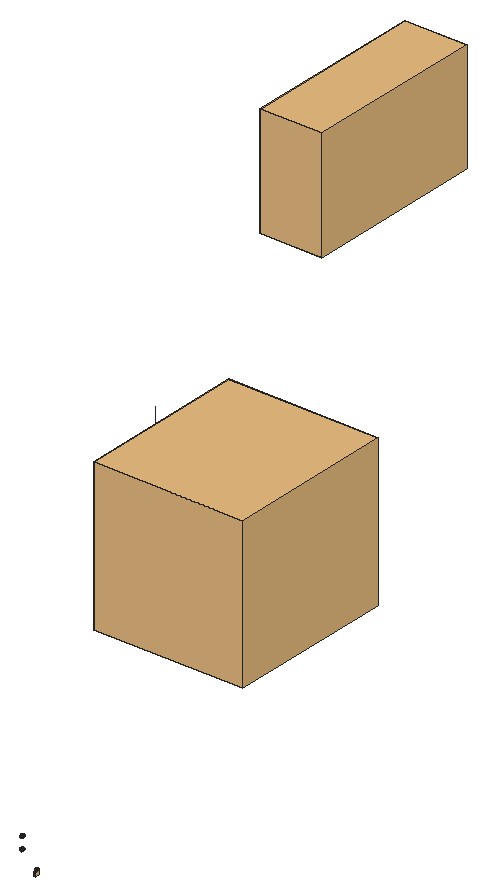
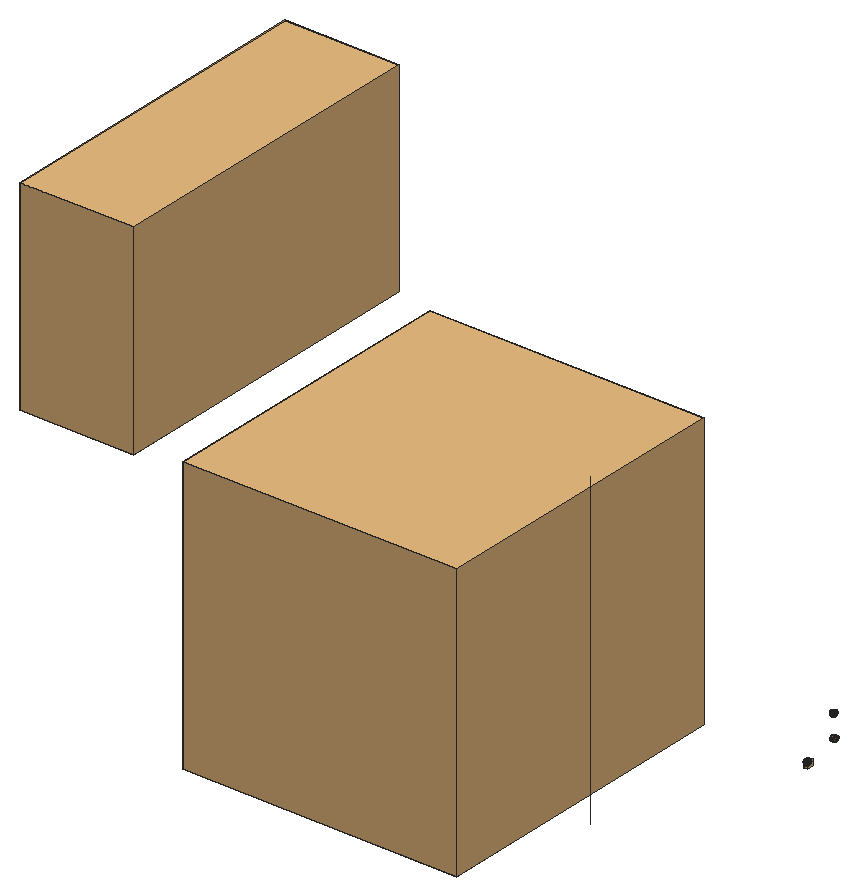
# SketchUp Ruby script. Lengths in inches.
U = 1.inch
M = Sketchup.active_model
def pt(a) = Geom::Point3d.new(a.map { |v| v * U })
def face(e, loops, mat)
  f = e.add_face(loops[0].map { |a| pt(a) })
  loops[1..].each { |l| e.add_face(l.map { |a| pt(a) }).erase! }
  f.material = f.back_material = mat if mat
  f
end
# faces: each face lists its corners as indices into pts; further lists are holes
def faces(e, pts, list, mat = nil) = list.each { |f| face(e, (f[0].is_a?(Array) ? f : [f]).map { |l| l.map { |i| pts[i] } }, mat) }
# xy, xz, yz: faces in a plane at the given z, y or x. An outline is a flat list of corners, or four numbers for a rectangle; further outlines are holes
def ring(l) = l.size == 4 ? [[l[0], l[1]], [l[2], l[1]], [l[2], l[3]], [l[0], l[3]]] : l.each_slice(2).to_a
def flat(e, list, mat, &to3) = list.each { |f| face(e, (f[0].is_a?(Array) ? f : [f]).map { |l| ring(l).map { |u, v| to3.(u, v) } }, mat) }
def xy(e, z, list, mat = nil) = flat(e, list, mat) { |x, y| [x, y, z] }
def xz(e, y, list, mat = nil) = flat(e, list, mat) { |x, z| [x, y, z] }
def yz(e, x, list, mat = nil) = flat(e, list, mat) { |y, z| [x, y, z] }
def lines(e, pts, list) = list.each { |a, b| e.add_line(pt(pts[a]), pt(pts[b])) }
# prism: a flat outline (further loops are holes) pulled along v
def prism(e, loops, v, mat = nil)
  f = face(e, loops, mat); d = Geom::Vector3d.new(v.map { |x| x * U })
  f.pushpull(f.normal.samedirection?(d) ? d.length : -d.length)
end
def box(e, o, s, mat = nil) = prism(e, [[o, [o[0] + s[0], o[1], o[2]], [o[0] + s[0], o[1] + s[1], o[2]], [o[0], o[1] + s[1], o[2]]]], [0, 0, s[2]], mat)
def at(x, y, z, deg = 0) = Geom::Transformation.translation(pt([x, y, z])) * Geom::Transformation.rotation(ORIGIN, Z_AXIS, deg.degrees)
def axes(o, x, y, z) = Geom::Transformation.new([*x, 0, *y, 0, *z, 0, *pt(o).to_a, 1])
def part(name) = M.definitions.add(name)
# library, detail: a bought-in or finely detailed component or shape, given as its bounding box
def library(name, o, s) = part(name).tap { |d| box(d.entities, o, s) }
def detail(e, o, s) = box(e.add_group.entities, o, s)
def put(e, d, t, mat = nil) = e.add_instance(d, t).tap { |i| i.material = mat if mat }
def group(e, t, mat = nil) = e.add_group.tap { |g| g.transformation = t; g.material = mat if mat }.entities
root = M.entities
M.materials.add("green").color = [174, 139, 102]
M.materials.add("vio").color = [206, 114, 100]
c1 = part("3DGeom~232_Defintion")
p = [[-0.24,-111.46,-482.48],[-247.71,40.8125,-431.68],[-3.37,-2.64,-500],[241.88,-45.39,-434.35],[50.53,96.35,-484.34],[-154.36,212.27,-404.56],
  [147.01,158.99,-439.69],[12.76,320.76,-327.23],[59.09,-200.9375,-436.46],[-242.29,-147.66,-401.33],[260.24,168.49,-378.02],[208.87,337.23,-220.41],
  [208.87,337.23,-220.41],[-139.53,-302.65,-321.625],[158.71,-247.11,-374.29],[271.93,-237.61,-312.62],[368.42,-174.96,-267.97],[422.32,-75.98,-252.31],
  [419.18,32.84,-269.83],[359.86,122.32,-315.85],[-242.29,-147.66,-401.33],[-425.69,73.33,-247.69],[-247.71,40.8125,-431.68],[-425.69,73.33,-247.69],
  [-317.89,271.31,-216.375],[-317.89,271.31,-216.375],[-154.36,212.27,-404.56],[-317.89,271.31,-216.375],[-124.92,396.59,-127.08],[-154.36,212.27,-404.56],
  [12.76,320.76,-327.23],[-139.53,-302.65,-321.625],[-419.42,-144.29,-212.64],[-242.29,-147.66,-401.33],[-242.29,-147.66,-401.33],[-425.69,73.33,-247.69],
  [260.24,168.49,-378.02],[381.41,257.26,-112.72],[359.86,122.32,-315.85],[260.24,168.49,-378.02],[208.87,337.23,-220.41],[33.01,-382.62,-213.94],
  [271.93,-237.61,-312.62],[33.01,-382.62,-213.94],[158.71,-247.11,-374.29],[12.76,320.76,-327.23],[101.53,415.61,-3.73],[12.76,320.76,-327.23],
  [208.87,337.23,-220.41],[33.01,-382.62,-213.94],[-300.77,-323.26,-120.61],[-139.53,-302.65,-321.625],[-139.53,-302.65,-321.625],[-300.77,-323.26,-120.61],
  [359.86,122.32,-315.85],[484.17,102.27,-33.02],[419.18,32.84,-269.83],[359.86,122.32,-315.85],[271.93,-237.61,-312.62],[229.12,-366.15,-107.12],
  [33.01,-382.62,-213.94],[368.42,-174.96,-267.97],[229.12,-366.15,-107.12],[271.93,-237.61,-312.62],[419.18,32.84,-269.83],[489.59,-86.2,-2.67],
  [419.18,32.84,-269.83],[422.32,-75.98,-252.31],[368.42,-174.96,-267.97],[396.24,-257.66,-29.79],[229.12,-366.15,-107.12],[422.32,-75.98,-252.31],
  [368.42,-174.96,-267.97],[422.32,-75.98,-252.31],[-489.59,86.2,2.67],[-425.69,73.33,-247.69],[-425.69,73.33,-247.69],[-396.24,257.66,29.79],
  [-425.69,73.33,-247.69],[-396.24,257.66,29.79],[-317.89,271.31,-216.375],[208.87,337.23,-220.41],[300.77,323.26,120.61],[381.41,257.26,-112.72],
  [208.87,337.23,-220.41],[300.77,323.26,120.61],[-396.24,257.66,29.79],[-229.12,366.15,107.12],[33.01,-382.62,-213.94],[-101.53,-415.61,3.73],
  [-300.77,-323.26,-120.61],[33.01,-382.62,-213.94],[-484.17,-102.27,33.02],[-33.01,382.62,213.94],[-381.41,-257.26,112.72],[-300.77,-323.26,-120.61],
  [-381.41,-257.26,112.72],[419.42,144.29,212.64],[300.77,323.26,120.61],[124.92,-396.59,127.08],[396.24,-257.66,-29.79],[425.69,-73.33,247.69],
  [396.24,-257.66,-29.79],[317.89,-271.31,216.375],[317.89,-271.31,216.375],[139.53,302.65,321.625],[139.53,302.65,321.625],[300.77,323.26,120.61],
  [-422.32,75.98,252.31],[-368.42,174.96,267.97],[-396.24,257.66,29.79],[-208.87,-337.23,220.41],[-381.41,-257.26,112.72],[-396.24,257.66,29.79],
  [-271.93,237.61,312.62],[-396.24,257.66,29.79],[-271.93,237.61,312.62],[-229.12,366.15,107.12],[-419.18,-32.84,269.83],[-271.93,237.61,312.62],
  [-158.71,247.11,374.29],[-158.71,247.11,374.29],[-208.87,-337.23,220.41],[-359.86,-122.32,315.85],[242.29,147.66,401.33],[139.53,302.65,321.625],
  [-12.76,-320.76,327.23],[317.89,-271.31,216.375],[247.71,-40.8125,431.68],[247.71,-40.8125,431.68],[-33.01,382.62,213.94],[-158.71,247.11,374.29],
  [-59.09,200.94,436.46],[-33.01,382.62,213.94],[139.53,302.65,321.625],[317.89,-271.31,216.375],[154.36,-212.27,404.56],[425.69,-73.33,247.69],
  [154.36,-212.27,404.56],[317.89,-271.31,216.375],[-208.87,-337.23,220.41],[-260.24,-168.49,378.02],[-12.76,-320.76,327.23],[-260.24,-168.49,378.02],
  [-208.87,-337.23,220.41],[425.69,-73.33,247.69],[247.71,-40.8125,431.68],[-422.32,75.98,252.31],[-419.18,-32.84,269.83],[-241.88,45.39,434.35],
  [-368.42,174.96,267.97],[-422.32,75.98,252.31],[-271.93,237.61,312.62],[-368.42,174.96,267.97],[-419.18,-32.84,269.83],[-359.86,-122.32,315.85],
  [-271.93,237.61,312.62],[-359.86,-122.32,315.85],[-260.24,-168.49,378.02],[139.53,302.65,321.625],[0.24,111.46,482.48],[139.53,302.65,321.625],
  [242.29,147.66,401.33],[-12.76,-320.76,327.23],[-147.01,-158.99,439.69],[-260.24,-168.49,378.02],[-12.76,-320.76,327.23],[-260.24,-168.49,378.02],
  [242.29,147.66,401.33],[3.37,2.64,500],[242.29,147.66,401.33],[-50.53,-96.35,484.34]]
faces(c1.entities,p,[[0,1,2],[0,2,3],[2,4,3],[2,1,5],[2,5,4],[4,6,3],[4,5,7],[4,7,6],
  [8,9,0],[8,0,3],[0,9,1],[6,10,3],[6,7,11],[6,12,10],[8,13,9],[14,13,8],
  [14,8,3],[15,14,3],[16,15,3],[17,16,3],[18,17,3],[19,18,3],[10,19,3],[20,21,22],
  [1,23,24],[1,25,5],[26,27,28],[29,28,30],[31,32,33],[34,32,35],[36,37,38],[39,40,37],
  [14,41,13],[42,43,44],[45,28,46],[47,46,48],[49,50,51],[52,53,32],[54,55,56],[57,37,55],
  [58,59,60],[61,62,63],[64,55,65],[66,65,67],[68,69,70],[71,69,72],[73,65,69],[32,74,75],
  [76,74,77],[78,79,80],[81,82,83],[84,46,85],[27,86,87],[27,87,28],[88,89,90],[59,89,91],
  [53,92,32],[32,92,74],[28,87,93],[28,93,46],[89,94,95],[53,96,92],[37,97,55],[37,98,97],
  [59,99,89],[100,99,59],[55,101,65],[55,97,101],[102,103,99],[65,104,69],[46,93,105],[46,106,107],
  [65,101,104],[92,108,74],[74,108,109],[74,109,110],[89,111,112],[99,111,89],[113,109,114],[115,116,117],
  [96,118,92],[92,118,108],[87,119,120],[87,121,93],[122,123,96],[96,123,118],[98,124,97],[98,125,124],
  [99,126,111],[127,126,99],[97,128,101],[97,124,129],[130,131,132],[133,132,134],[135,136,126],[137,138,139],
  [140,141,123],[142,143,144],[145,146,138],[147,148,149],[150,151,149],[152,153,149],[154,155,149],[131,156,149],
  [157,158,149],[159,132,160],[161,160,162],[163,164,165],[138,164,166],[132,131,149],[167,164,149],[168,169,146],
  [170,160,169],[138,171,164],[146,171,138],[146,169,171],[164,171,149],[171,169,149],[169,160,149],[160,132,149]],"vio")
c2 = part("3DGeom~234_Defintion")
p = [[-0.24,-111.46,-482.48],[-247.71,40.8125,-431.68],[-3.37,-2.64,-500],[241.88,-45.39,-434.35],[50.53,96.35,-484.34],[-154.36,212.27,-404.56],
  [147.01,158.99,-439.69],[12.76,320.76,-327.23],[59.09,-200.9375,-436.46],[-242.29,-147.66,-401.33],[260.24,168.49,-378.02],[208.87,337.23,-220.41],
  [208.87,337.23,-220.41],[-139.53,-302.65,-321.625],[158.71,-247.11,-374.29],[271.93,-237.61,-312.62],[368.42,-174.96,-267.97],[422.32,-75.98,-252.31],
  [419.18,32.84,-269.83],[359.86,122.32,-315.85],[-242.29,-147.66,-401.33],[-425.69,73.33,-247.69],[-247.71,40.8125,-431.68],[-425.69,73.33,-247.69],
  [-317.89,271.31,-216.375],[-317.89,271.31,-216.375],[-154.36,212.27,-404.56],[-317.89,271.31,-216.375],[-124.92,396.59,-127.08],[-154.36,212.27,-404.56],
  [12.76,320.76,-327.23],[-139.53,-302.65,-321.625],[-419.42,-144.29,-212.64],[-242.29,-147.66,-401.33],[-242.29,-147.66,-401.33],[-425.69,73.33,-247.69],
  [260.24,168.49,-378.02],[381.41,257.26,-112.72],[359.86,122.32,-315.85],[260.24,168.49,-378.02],[208.87,337.23,-220.41],[33.01,-382.62,-213.94],
  [271.93,-237.61,-312.62],[33.01,-382.62,-213.94],[158.71,-247.11,-374.29],[12.76,320.76,-327.23],[101.53,415.61,-3.73],[12.76,320.76,-327.23],
  [208.87,337.23,-220.41],[33.01,-382.62,-213.94],[-300.77,-323.26,-120.61],[-139.53,-302.65,-321.625],[-139.53,-302.65,-321.625],[-300.77,-323.26,-120.61],
  [359.86,122.32,-315.85],[484.17,102.27,-33.02],[419.18,32.84,-269.83],[359.86,122.32,-315.85],[271.93,-237.61,-312.62],[229.12,-366.15,-107.12],
  [33.01,-382.62,-213.94],[368.42,-174.96,-267.97],[229.12,-366.15,-107.12],[271.93,-237.61,-312.62],[419.18,32.84,-269.83],[489.59,-86.2,-2.67],
  [419.18,32.84,-269.83],[422.32,-75.98,-252.31],[368.42,-174.96,-267.97],[396.24,-257.66,-29.79],[229.12,-366.15,-107.12],[422.32,-75.98,-252.31],
  [368.42,-174.96,-267.97],[422.32,-75.98,-252.31],[-489.59,86.2,2.67],[-425.69,73.33,-247.69],[-425.69,73.33,-247.69],[-396.24,257.66,29.79],
  [-425.69,73.33,-247.69],[-396.24,257.66,29.79],[-317.89,271.31,-216.375],[208.87,337.23,-220.41],[300.77,323.26,120.61],[381.41,257.26,-112.72],
  [208.87,337.23,-220.41],[300.77,323.26,120.61],[-396.24,257.66,29.79],[-229.12,366.15,107.12],[33.01,-382.62,-213.94],[-101.53,-415.61,3.73],
  [-300.77,-323.26,-120.61],[33.01,-382.62,-213.94],[-484.17,-102.27,33.02],[-33.01,382.62,213.94],[-381.41,-257.26,112.72],[-300.77,-323.26,-120.61],
  [-381.41,-257.26,112.72],[419.42,144.29,212.64],[300.77,323.26,120.61],[124.92,-396.59,127.08],[396.24,-257.66,-29.79],[425.69,-73.33,247.69],
  [396.24,-257.66,-29.79],[317.89,-271.31,216.375],[317.89,-271.31,216.375],[139.53,302.65,321.625],[139.53,302.65,321.625],[300.77,323.26,120.61],
  [-422.32,75.98,252.31],[-368.42,174.96,267.97],[-396.24,257.66,29.79],[-208.87,-337.23,220.41],[-381.41,-257.26,112.72],[-396.24,257.66,29.79],
  [-271.93,237.61,312.62],[-396.24,257.66,29.79],[-271.93,237.61,312.62],[-229.12,366.15,107.12],[-419.18,-32.84,269.83],[-271.93,237.61,312.62],
  [-158.71,247.11,374.29],[-158.71,247.11,374.29],[-208.87,-337.23,220.41],[-359.86,-122.32,315.85],[242.29,147.66,401.33],[139.53,302.65,321.625],
  [-12.76,-320.76,327.23],[317.89,-271.31,216.375],[247.71,-40.8125,431.68],[247.71,-40.8125,431.68],[-33.01,382.62,213.94],[-158.71,247.11,374.29],
  [-59.09,200.94,436.46],[-33.01,382.62,213.94],[139.53,302.65,321.625],[317.89,-271.31,216.375],[154.36,-212.27,404.56],[425.69,-73.33,247.69],
  [154.36,-212.27,404.56],[317.89,-271.31,216.375],[-208.87,-337.23,220.41],[-260.24,-168.49,378.02],[-12.76,-320.76,327.23],[-260.24,-168.49,378.02],
  [-208.87,-337.23,220.41],[425.69,-73.33,247.69],[247.71,-40.8125,431.68],[-422.32,75.98,252.31],[-419.18,-32.84,269.83],[-241.88,45.39,434.35],
  [-368.42,174.96,267.97],[-422.32,75.98,252.31],[-271.93,237.61,312.62],[-368.42,174.96,267.97],[-419.18,-32.84,269.83],[-359.86,-122.32,315.85],
  [-271.93,237.61,312.62],[-359.86,-122.32,315.85],[-260.24,-168.49,378.02],[139.53,302.65,321.625],[0.24,111.46,482.48],[139.53,302.65,321.625],
  [242.29,147.66,401.33],[-12.76,-320.76,327.23],[-147.01,-158.99,439.69],[-260.24,-168.49,378.02],[-12.76,-320.76,327.23],[-260.24,-168.49,378.02],
  [242.29,147.66,401.33],[3.37,2.64,500],[242.29,147.66,401.33],[-50.53,-96.35,484.34]]
faces(c2.entities,p,[[0,1,2],[0,2,3],[2,4,3],[2,1,5],[2,5,4],[4,6,3],[4,5,7],[4,7,6],
  [8,9,0],[8,0,3],[0,9,1],[6,10,3],[6,7,11],[6,12,10],[8,13,9],[14,13,8],
  [14,8,3],[15,14,3],[16,15,3],[17,16,3],[18,17,3],[19,18,3],[10,19,3],[20,21,22],
  [1,23,24],[1,25,5],[26,27,28],[29,28,30],[31,32,33],[34,32,35],[36,37,38],[39,40,37],
  [14,41,13],[42,43,44],[45,28,46],[47,46,48],[49,50,51],[52,53,32],[54,55,56],[57,37,55],
  [58,59,60],[61,62,63],[64,55,65],[66,65,67],[68,69,70],[71,69,72],[73,65,69],[32,74,75],
  [76,74,77],[78,79,80],[81,82,83],[84,46,85],[27,86,87],[27,87,28],[88,89,90],[59,89,91],
  [53,92,32],[32,92,74],[28,87,93],[28,93,46],[89,94,95],[53,96,92],[37,97,55],[37,98,97],
  [59,99,89],[100,99,59],[55,101,65],[55,97,101],[102,103,99],[65,104,69],[46,93,105],[46,106,107],
  [65,101,104],[92,108,74],[74,108,109],[74,109,110],[89,111,112],[99,111,89],[113,109,114],[115,116,117],
  [96,118,92],[92,118,108],[87,119,120],[87,121,93],[122,123,96],[96,123,118],[98,124,97],[98,125,124],
  [99,126,111],[127,126,99],[97,128,101],[97,124,129],[130,131,132],[133,132,134],[135,136,126],[137,138,139],
  [140,141,123],[142,143,144],[145,146,138],[147,148,149],[150,151,149],[152,153,149],[154,155,149],[131,156,149],
  [157,158,149],[159,132,160],[161,160,162],[163,164,165],[138,164,166],[132,131,149],[167,164,149],[168,169,146],
  [170,160,169],[138,171,164],[146,171,138],[146,169,171],[164,171,149],[171,169,149],[169,160,149],[160,132,149]],"vio")
c3 = library("3DGeom~57_Defintion",[-500,-478.45,-265.375],[1000,956.89,530.75])
c4 = part("3DGeom~58_Defintion")
p = [[-465.47,464.9,-258.6875],[-477.89,451.53,-263.24],[-489.74,438.22,-257.15],[-465.47,464.9,-258.6875],[-497.83,428.53,-242.0625],[-500,425.07,-222.01],
  [-465.47,464.9,-258.6875],[-500,425.07,-222.01],[-495.67,428.76,-202.375],[-465.47,464.9,-258.6875],[-489.74,438.22,-257.15],[-497.83,428.53,-242.0625],
  [-465.47,464.9,-258.6875],[-495.67,428.76,-202.375],[-485.99,438.61,-188.41],[-465.47,464.9,-258.6875],[-485.99,438.61,-188.41],[-473.5625,451.98,-183.86],
  [-465.47,464.9,-258.6875],[-473.5625,451.98,-183.86],[-461.72,465.3,-189.95],[-465.47,464.9,-258.6875],[-453.625,474.98,-205.04],[-451.46,478.44,-225.09],
  [-465.47,464.9,-258.6875],[-451.46,478.44,-225.09],[-455.79,474.75,-244.72],[-465.47,464.9,-258.6875],[-461.72,465.3,-189.95],[-453.625,474.98,-205.04],
  [492.22,-453.97,197.65],[460.87,-474.71,197.28],[477.9,-465.75,192.59],[460.87,-474.71,197.28],[436.46,-475.96,228.62],[445.7,-478.45,210.47],
  [460.87,-474.71,197.28],[492.22,-453.97,197.65],[436.46,-475.96,228.62],[436.46,-475.96,228.62],[492.22,-453.97,197.65],[443.4,-456.48,260.3125],
  [443.4,-456.48,260.3125],[492.22,-453.97,197.65],[474.74,-435.74,260.68],[474.74,-435.74,260.68],[492.22,-453.97,197.65],[499.15,-434.48,229.35],
  [492.22,-453.97,197.65],[500,-442.52,211.1],[499.15,-434.48,229.35],[436.46,-475.96,228.62],[443.4,-456.48,260.3125],[435.61,-467.92,246.86],
  [474.74,-435.74,260.68],[499.15,-434.48,229.35],[489.91,-432,247.49],[443.4,-456.48,260.3125],[474.74,-435.74,260.68],[457.72,-444.7,265.375]]
faces(c4.entities,p,[[0,1,2],[3,4,5],[6,7,8],[9,10,11],[12,13,14],[15,16,17],[18,19,20],[21,22,23],
  [24,25,26],[27,28,29],[30,31,32],[33,34,35],[36,37,38],[39,40,41],[42,43,44],[45,46,47],
  [48,49,50],[51,52,53],[54,55,56],[57,58,59]],"green")
c5 = part("3DGeom~204_Defintion")
p = [[-12.5,-12.78,-500],[-167.87,-176.1875,-423.23],[-275,-119.8,-393.5],[139.12,-146.19,-448.74],[321.29,0,-383.61],[-198.05,84.89,-448.51],
  [146.22,154.06,-442.79],[216.18,-279.61,-308.47],[-80.33,-253.22,-393.64],[410.28,-154.06,-221.63],[410.28,-154.06,-221.63],[-373.01,-99.16,-312.41],
  [-373.01,-99.16,-312.41],[-367.81,120.64,-308.0625],[-68.03,266.84,-383.34],[-367.81,120.64,-308.0625],[-68.03,266.84,-383.34],[417.375,146.19,-215.68],
  [417.375,146.19,-215.68],[265.76,279.61,-266.94],[265.76,279.61,-266.94],[-68.03,266.84,-383.34],[-278.26,-292.39,-233.06],[-278.26,-292.39,-233.06],
  [-35.84,-330.25,-312.65],[-278.26,-292.39,-233.06],[-373.01,-99.16,-312.41],[-275,-119.8,-393.5],[-278.26,-292.39,-233.06],[494.4375,12.78,-75.41],
  [410.28,-154.06,-221.63],[321.29,0,-383.61],[321.29,0,-383.61],[417.375,146.19,-215.68],[-68.03,266.84,-383.34],[-367.81,120.64,-308.0625],
  [-264.06,308.11,-221.16],[80.21,377.28,-215.45],[-68.03,266.84,-383.34],[-264.06,308.11,-221.16],[265.76,279.61,-266.94],[-68.03,266.84,-383.34],
  [80.21,377.28,-215.45],[-35.84,-330.25,-312.65],[-46.32,-386.64,-201.97],[-278.26,-292.39,-233.06],[198.04,-377.28,-116.76],[-35.84,-330.25,-312.65],
  [198.04,-377.28,-116.76],[-35.84,-330.25,-312.65],[216.18,-279.61,-308.47],[-435.64,-119.8,-201.7],[-278.26,-292.39,-233.06],[-367.81,120.64,-308.0625],
  [389.33,-266.84,-0.27],[198.04,-377.28,-116.76],[216.18,-279.61,-308.47],[216.18,-279.61,-308.47],[-476.3,84.89,-116.29],[-264.06,308.11,-221.16],
  [401.625,253.22,10.03],[265.76,279.61,-266.94],[265.76,279.61,-266.94],[314.09,330.25,-19.5625],[314.09,330.25,-19.5625],[265.76,279.61,-266.94],
  [-108.95,-407.27,-91.25],[-206.96,-386.64,-10.17],[-314.09,-330.25,19.5625],[-314.09,-330.25,19.5625],[-401.625,-253.22,-10.03],[-278.26,-292.39,-233.06],
  [-446.12,-176.1875,-91.02],[-278.26,-292.39,-233.06],[-278.26,-292.39,-233.06],[476.3,-84.89,116.29],[-264.06,308.11,-221.16],[-389.33,266.84,0.27],
  [-89.55,413.03,-75],[-389.33,266.84,0.27],[446.12,176.1875,91.02],[206.96,386.64,10.17],[89.55,-413.03,75],[198.04,-377.28,-116.76],
  [264.06,-308.11,221.16],[198.04,-377.28,-116.76],[264.06,-308.11,221.16],[198.04,-377.28,-116.76],[389.33,-266.84,-0.27],[-494.4375,-12.78,75.41],
  [-80.21,-377.28,215.45],[435.64,119.8,201.7],[-389.33,266.84,0.27],[-198.04,377.28,116.76],[108.95,407.27,91.25],[314.09,330.25,-19.5625],
  [278.26,292.39,233.06],[278.26,292.39,233.06],[-265.76,-279.61,266.94],[-265.76,-279.61,266.94],[-417.375,-146.19,215.68],[-314.09,-330.25,19.5625],
  [-417.375,-146.19,215.68],[367.81,-120.64,308.0625],[264.06,-308.11,221.16],[367.81,-120.64,308.0625],[-410.28,154.06,221.63],[-198.04,377.28,116.76],
  [-410.28,154.06,221.63],[278.26,292.39,233.06],[-417.375,-146.19,215.68],[-314.09,-330.25,19.5625],[-265.76,-279.61,266.94],[68.03,-266.84,383.34],
  [68.03,-266.84,383.34],[264.06,-308.11,221.16],[-410.28,154.06,221.63],[-417.375,-146.19,215.68],[46.32,386.64,201.97],[278.26,292.39,233.06],
  [373.01,99.16,312.41],[367.81,-120.64,308.0625],[-198.04,377.28,116.76],[-410.28,154.06,221.63],[-216.18,279.61,308.47],[-216.18,279.61,308.47],
  [-216.18,279.61,308.47],[35.84,330.25,312.65],[35.84,330.25,312.65],[278.26,292.39,233.06],[-146.22,-154.06,442.79],[-265.76,-279.61,266.94],
  [-80.21,-377.28,215.45],[-80.21,-377.28,215.45],[68.03,-266.84,383.34],[-321.29,0,383.61],[-417.375,-146.19,215.68],[-410.28,154.06,221.63],
  [-417.375,-146.19,215.68],[-321.29,0,383.61],[198.05,-84.89,448.51],[264.06,-308.11,221.16],[367.81,-120.64,308.0625],[-216.18,279.61,308.47],
  [-410.28,154.06,221.63],[275,119.8,393.5],[167.87,176.1875,423.23],[275,119.8,393.5],[278.26,292.39,233.06],[80.33,253.22,393.64],
  [278.26,292.39,233.06],[35.84,330.25,312.65],[278.26,292.39,233.06],[275,119.8,393.5],[275,119.8,393.5],[373.01,99.16,312.41],
  [-139.12,146.19,448.74],[12.5,12.78,500],[275,119.8,393.5]]
faces(c5.entities,p,[[0,1,2],[3,1,0],[4,3,0],[0,2,5],[6,0,5],[4,0,6],[7,8,3],[9,7,3],
  [3,8,1],[10,3,4],[5,2,11],[5,12,13],[14,5,15],[6,5,16],[17,4,6],[18,6,19],
  [20,6,21],[2,1,22],[1,8,23],[8,24,25],[7,24,8],[26,27,28],[29,30,31],[29,32,33],
  [34,35,36],[37,38,39],[40,41,42],[43,44,45],[46,44,47],[48,49,50],[51,26,52],[53,26,51],
  [54,55,56],[54,57,30],[53,51,58],[59,53,58],[60,33,61],[60,62,63],[64,65,37],[66,67,45],
  [44,66,45],[67,68,45],[69,70,71],[70,72,73],[72,51,74],[75,54,30],[75,30,29],[76,58,77],
  [78,39,79],[37,39,78],[80,29,33],[80,33,60],[64,37,81],[81,37,78],[82,66,44],[82,44,83],
  [58,51,72],[84,82,85],[86,87,88],[58,72,89],[77,58,89],[90,66,82],[90,67,66],[89,72,70],
  [91,75,29],[91,29,80],[78,92,93],[94,78,93],[81,78,94],[60,95,96],[64,81,97],[98,68,67],
  [99,67,90],[100,70,101],[89,70,102],[103,104,54],[105,54,75],[77,89,106],[107,77,108],[80,60,96],
  [81,94,109],[110,111,112],[113,90,82],[114,82,115],[116,89,117],[91,80,96],[94,118,119],[94,93,118],
  [120,121,75],[120,75,91],[122,123,124],[118,93,125],[120,91,96],[118,126,127],[118,128,129],[130,131,132],
  [130,133,134],[135,136,131],[137,138,139],[140,134,141],[140,141,142],[143,144,135],[145,120,96],[146,147,148],
  [149,146,150],[151,149,152],[135,131,130],[153,140,142],[154,142,155],[143,135,156],[151,143,156],[151,156,149],
  [157,130,134],[157,134,140],[156,135,130],[146,140,158],[149,156,157],[149,157,146],[146,157,140],[156,130,157]],"vio")
c6 = library("ceramic vase with flowers",[-9.61,-11.6875,0],[28.98,26,22.72])
c7 = library("flowers vase",[13.94,34.08,0],[79.78,27.28,49.07])
p = [[6,162,66],[6,162,48]]
lines(root,p,[[0,1]])
g1 = group(root,at(15.3125,134.49,26.21))
put(g1,c1,axes([-2.06,0.89,13.3],[0,0.00039,0],[0,0,-0.00039],[-0.00039,0,0]),"vio")
g2 = group(root,at(15.3125,134.49,26.21))
put(g2,c2,axes([-2.11,0.91,12.02],[0,0.00039,0],[0,0,-0.00039],[-0.00039,0,0]),"vio")
g3 = group(root,at(15.3125,134.49,26.21))
put(g3,c3,axes([-0.65,0.96,10.24],[0,0.00037,0],[0,0,-0.00037],[-0.00037,0,0]),"green")
put(g3,c4,axes([-0.65,0.96,10.24],[0,0.00037,0],[0,0,-0.00037],[-0.00037,0,0]),"green")
g4 = group(root,at(15.3125,134.49,26.21))
put(g4,c5,axes([-0.75,1.16,10.43],[0,0.00039,0],[0,0,-0.00039],[-0.00039,0,0]),"vio")
put(root,c6,axes([15.33,159,49],[0,0.61641,0],[-0.609,0,0],[0,0,0.7]))
put(root,c7,axes([0.77,168.875,79],[0,0.24,0],[0.24,0,0],[0,0,0.24]))
